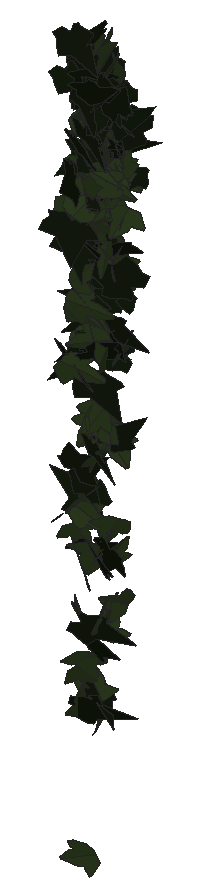
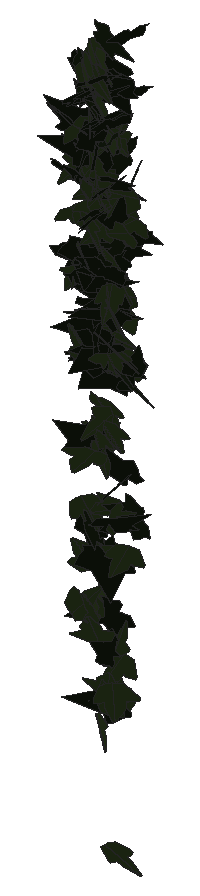
# SketchUp Ruby script. Lengths in inches.
U = 1.inch
M = Sketchup.active_model
def pt(a) = Geom::Point3d.new(a.map { |v| v * U })
def face(e, loops, mat)
  f = e.add_face(loops[0].map { |a| pt(a) })
  loops[1..].each { |l| e.add_face(l.map { |a| pt(a) }).erase! }
  f.material = f.back_material = mat if mat
  f
end
# faces: each face lists its corners as indices into pts; further lists are holes
def faces(e, pts, list, mat = nil) = list.each { |f| face(e, (f[0].is_a?(Array) ? f : [f]).map { |l| l.map { |i| pts[i] } }, mat) }
# xy, xz, yz: faces in a plane at the given z, y or x. An outline is a flat list of corners, or four numbers for a rectangle; further outlines are holes
def ring(l) = l.size == 4 ? [[l[0], l[1]], [l[2], l[1]], [l[2], l[3]], [l[0], l[3]]] : l.each_slice(2).to_a
def flat(e, list, mat, &to3) = list.each { |f| face(e, (f[0].is_a?(Array) ? f : [f]).map { |l| ring(l).map { |u, v| to3.(u, v) } }, mat) }
def xy(e, z, list, mat = nil) = flat(e, list, mat) { |x, y| [x, y, z] }
def xz(e, y, list, mat = nil) = flat(e, list, mat) { |x, z| [x, y, z] }
def yz(e, x, list, mat = nil) = flat(e, list, mat) { |y, z| [x, y, z] }
def lines(e, pts, list) = list.each { |a, b| e.add_line(pt(pts[a]), pt(pts[b])) }
# prism: a flat outline (further loops are holes) pulled along v
def prism(e, loops, v, mat = nil)
  f = face(e, loops, mat); d = Geom::Vector3d.new(v.map { |x| x * U })
  f.pushpull(f.normal.samedirection?(d) ? d.length : -d.length)
end
def box(e, o, s, mat = nil) = prism(e, [[o, [o[0] + s[0], o[1], o[2]], [o[0] + s[0], o[1] + s[1], o[2]], [o[0], o[1] + s[1], o[2]]]], [0, 0, s[2]], mat)
def at(x, y, z, deg = 0) = Geom::Transformation.translation(pt([x, y, z])) * Geom::Transformation.rotation(ORIGIN, Z_AXIS, deg.degrees)
def axes(o, x, y, z) = Geom::Transformation.new([*x, 0, *y, 0, *z, 0, *pt(o).to_a, 1])
def part(name) = M.definitions.add(name)
# library, detail: a bought-in or finely detailed component or shape, given as its bounding box
def library(name, o, s) = part(name).tap { |d| box(d.entities, o, s) }
def detail(e, o, s) = box(e.add_group.entities, o, s)
def put(e, d, t, mat = nil) = e.add_instance(d, t).tap { |i| i.material = mat if mat }
def group(e, t, mat = nil) = e.add_group.tap { |g| g.transformation = t; g.material = mat if mat }.entities
root = M.entities
M.materials.add("1026 AP 7946 SUNNY SIDE UP").color = [254, 231, 186]
M.materials.add("efeu1").color = [18, 25, 13]
M.materials.add("efeu2").color = [43, 57, 29]
c1 = part("ivyleaf_10")
p = [[0,0.5,-0.03],[-0.0625,2.02,-0.43],[-0.19,2.01,-0.46],[-0.54,1.05,-0.29],[-0.52,0.625,-0.18],[-0.83,0.76,-0.28],
  [-1.16,0.64,-0.33],[-1.15,0.33,-0.24],[-0.77,-0.39,0.02],[-0.3,-0.51,0.16],[0.04,-0.48,0.23],[-0.02,2.01,-0.4375],
  [-0.06,2.01,-0.43],[0.04,-0.49,0.23],[0.67,-0.49,0.14],[1.38,0.36,-0.2],[1.375,0.51,-0.24],[0.81,0.65,-0.19],
  [0.62,0.59,-0.15],[0.6,1.09,-0.28],[0.5,1.23,-0.31]]
faces(c1.entities,p,[[0,1,2,3,4,5,6,7,8,9,10],[11,12,0,13,14,15,16,17,18,19,20]],"efeu2")
c2 = part("ivyleaf_9")
p = [[1.54,2.16,1.25],[1.36,2.04,1.19],[-0.21,0.99,0.68],[-0.71,1.11,0.82],[-0.85,0.86,0.67],[-0.8,0.17,0.21],
  [-0.9,-0.01,0.1],[-0.67,-0.16,-0.02],[-0.08,-0.08,-0.05],[-0.03,-0.6,-0.4],[0.65,-0.88,-0.66],[0.83,-0.6,-0.49],
  [1.29,-0.42,-0.43],[1.8125,-0.07,-0.26],[1.21,0.44,0.15]]
faces(c2.entities,p,[[0,1,2,3,4,5,6,7,8,9,10,11,12,13,14]],"efeu1")
put(root,c1,axes([112.32,212.58,262.16],[0.2763,-0.17067,-0.05977],[0.08284,-0.02746,0.25162],[-0.27056,-0.18269,0.016]),"1026 AP 7946 SUNNY SIDE UP")
put(root,c2,axes([112.64,212.18,261],[-0.35335,0.1338,-0.06385],[0.06641,-0.05128,-0.26879],[-0.22268,-0.22761,0.02116]),"1026 AP 7946 SUNNY SIDE UP")
put(root,c1,axes([112.42,212.25,257.27],[-0.22363,-0.16972,-0.11593],[0.13077,0.0756,-0.22725],[0.29137,-0.16419,0.01301]),"1026 AP 7946 SUNNY SIDE UP")
put(root,c1,axes([112.52,212.29,255.31],[-0.24576,0.18393,0.0036],[0.01054,0.00248,0.24858],[0.28905,0.1563,-0.006]),"1026 AP 7946 SUNNY SIDE UP")
put(root,c1,axes([112.53,212.48,254.42],[-0.26293,-0.21485,0.00041],[0.01833,-0.01112,-0.28005],[0.33734,-0.16685,0.01554]),"1026 AP 7946 SUNNY SIDE UP")
put(root,c2,axes([112.67,212.58,265.125],[-0.37632,-0.06247,0.0594],[-0.07698,-0.04082,-0.2536],[0.10975,-0.24285,0.02579]),"1026 AP 7946 SUNNY SIDE UP")
put(root,c2,axes([112.74,212.43,257.79],[-0.29869,-0.19911,-0.04621],[-0.05273,-0.02843,0.28329],[-0.31617,0.19284,-0.00359]),"1026 AP 7946 SUNNY SIDE UP")
put(root,c1,axes([112.34,212.1875,264.2],[-0.27957,-0.08913,-0.13707],[0.24883,-0.07137,-0.16966],[0.0341,-0.20996,0.11426]),"1026 AP 7946 SUNNY SIDE UP")
put(root,c1,axes([112.56,212.46,266.07],[0.03135,-0.22524,0.12427],[0.00019,-0.12227,-0.23346],[0.40271,0.01759,-0.00956]),"1026 AP 7946 SUNNY SIDE UP")
put(root,c2,axes([112.33,212.16,266.99],[0.09061,-0.19392,-0.16045],[0.07592,0.16449,-0.19301],[0.38255,0.01328,0.07631]),"1026 AP 7946 SUNNY SIDE UP")
put(root,c2,axes([112.48,211.77,257.76],[-0.06386,0.25255,-0.09168],[-0.0318,0.08831,0.26397],[0.42059,0.04503,0.00604]),"1026 AP 7946 SUNNY SIDE UP")
put(root,c2,axes([112.51,212.09,264.69],[-0.03269,-0.0761,0.28244],[-0.09868,-0.26734,-0.08279],[0.43705,-0.06605,0.00243]),"1026 AP 7946 SUNNY SIDE UP")
put(root,c2,axes([112.51,212.01,263.88],[-0.26999,-0.16735,-0.12115],[0.14648,0.07132,-0.24625],[0.28536,-0.19494,0.01178]),"1026 AP 7946 SUNNY SIDE UP")
put(root,c2,axes([112.77,212.51,261.75],[-0.34185,0.11338,-0.00493],[-0.00847,-0.02204,-0.2517],[-0.17828,-0.21635,0.02143]),"1026 AP 7946 SUNNY SIDE UP")
put(root,c1,axes([112.56,212.48,262.77],[-0.14162,-0.25149,-0.10523],[0.09043,0.08596,-0.27362],[0.41626,-0.10424,0.02364]),"1026 AP 7946 SUNNY SIDE UP")
put(root,c1,axes([112.27,212.35,264.83],[-0.0931,-0.0054,-0.26878],[0.39706,-0.06857,-0.05798],[-0.10334,-0.25857,0.01937]),"1026 AP 7946 SUNNY SIDE UP")
put(root,c2,axes([112.44,212.58,266.46],[0.04423,-0.2333,-0.12414],[-0.00425,0.11959,-0.24115],[0.41191,0.02629,0.01084]),"1026 AP 7946 SUNNY SIDE UP")
put(root,c1,axes([112.41,212.44,266.1],[0.07251,-0.14138,0.2086],[0.26726,-0.1323,-0.13529],[0.28314,0.16109,0.07427]),"1026 AP 7946 SUNNY SIDE UP")
put(root,c1,axes([112.34,212.38,264.0625],[0.23882,0.01083,0.20798],[0.31655,-0.03048,-0.15457],[0.02817,0.25074,-0.02628]),"1026 AP 7946 SUNNY SIDE UP")
put(root,c1,axes([112.66,212.3,257.89],[0.0368,0.03694,-0.25423],[-0.13133,-0.23263,-0.04536],[-0.37007,0.08623,-0.00918]),"1026 AP 7946 SUNNY SIDE UP")
put(root,c1,axes([112.59,212.35,264.58],[-0.07442,0.22567,-0.06463],[0.0126,-0.06372,-0.23786],[-0.36864,-0.04773,0.00492]),"1026 AP 7946 SUNNY SIDE UP")
put(root,c1,axes([112.65,212.4,264.57],[0.30029,0.12402,-0.07462],[-0.09595,-0.04031,-0.23482],[-0.20505,0.20048,0.00061]),"1026 AP 7946 SUNNY SIDE UP")
put(root,c1,axes([112.55,212.625,262.64],[-0.03571,0.10642,-0.25194],[0.06017,-0.24221,-0.11339],[-0.41591,-0.04418,0.00523]),"1026 AP 7946 SUNNY SIDE UP")
put(root,c2,axes([112.43,212.18,265.57],[0.30095,-0.21064,0.01925],[-0.00065,-0.02718,-0.29274],[0.33269,0.1905,-0.01798]),"1026 AP 7946 SUNNY SIDE UP")
put(root,c1,axes([112.65,212.43,261.37],[0.29796,0.14273,-0.06151],[-0.05722,-0.05195,-0.24391],[-0.23696,0.19202,-0.01845]),"1026 AP 7946 SUNNY SIDE UP")
put(root,c2,axes([112.39,212.06,260.9],[0.14027,-0.16506,0.24365],[0.13509,-0.22214,-0.19364],[0.43418,0.12244,-0.01847]),"1026 AP 7946 SUNNY SIDE UP")
put(root,c1,axes([112.54,212.3,266.01],[0.14169,0.20034,0.1309],[0.10074,0.10905,-0.22534],[-0.35818,0.10992,-0.0116]),"1026 AP 7946 SUNNY SIDE UP")
put(root,c2,axes([112.55,212.35,262.46],[0.02897,0.10758,-0.25264],[-0.0118,0.24653,0.11201],[0.42179,-0.00049,0.02048]),"1026 AP 7946 SUNNY SIDE UP")
put(root,c2,axes([112.62,212.16,263.49],[-0.17884,-0.2304,-0.06982],[0.05918,0.0555,-0.26422],[0.37238,-0.11947,0.00846]),"1026 AP 7946 SUNNY SIDE UP")
put(root,c2,axes([112.47,212.51,264.37],[-0.01172,-0.06513,0.25169],[0.1762,-0.22036,-0.0582],[0.35702,0.10662,0.03698]),"1026 AP 7946 SUNNY SIDE UP")
put(root,c2,axes([112.55,212.56,265.04],[0.08673,-0.24778,-0.04562],[-0.0048,0.04323,-0.26118],[0.39537,0.05488,0.00683]),"1026 AP 7946 SUNNY SIDE UP")
put(root,c2,axes([112.59,211.92,267.98],[0.08654,-0.23035,-0.15185],[-0.03314,0.145,-0.24286],[0.42762,0.05785,0.01191]),"1026 AP 7946 SUNNY SIDE UP")
put(root,c1,axes([112.69,212.52,263.6],[0.32967,-0.13557,0.05425],[0.0548,-0.04425,-0.25681],[0.22247,0.21179,-0.01713]),"1026 AP 7946 SUNNY SIDE UP")
put(root,c1,axes([112.61,212.07,264.14],[0.26202,0.07095,-0.16182],[0.18111,0.11742,0.18074],[0.20238,-0.19692,0.04776]),"1026 AP 7946 SUNNY SIDE UP")
put(root,c1,axes([112.75,212.55,267.6],[0.20593,-0.22152,0.04877],[0.01978,-0.04894,-0.26501],[0.35605,0.13084,-0.01348]),"1026 AP 7946 SUNNY SIDE UP")
put(root,c2,axes([112.95,212.375,261.3],[-0.0124,0.01839,-0.27797],[-0.09809,-0.26289,-0.01811],[-0.41396,0.06175,0.01262]),"1026 AP 7946 SUNNY SIDE UP")
put(root,c2,axes([112.9,212.26,267.06],[0.08514,0.13614,-0.21514],[-0.08235,-0.20353,-0.15131],[-0.38428,0.07378,-0.01524]),"1026 AP 7946 SUNNY SIDE UP")
put(root,c2,axes([112.85,212.25,257.03],[0.22671,0.19448,-0.12512],[-0.09876,-0.10583,-0.24976],[-0.3477,0.15687,-0.01064]),"1026 AP 7946 SUNNY SIDE UP")
put(root,c1,axes([113.08,212.52,267.28],[-0.272,0.06176,0.22464],[-0.349,0.00713,-0.18373],[-0.06939,-0.27797,0.04349]),"1026 AP 7946 SUNNY SIDE UP")
put(root,c2,axes([112.76,212.6,265.875],[-0.1826,-0.13166,0.20436],[0.02255,-0.22488,-0.14588],[0.37467,-0.05063,0.10838]),"1026 AP 7946 SUNNY SIDE UP")
put(root,c2,axes([112.77,212.32,262.7],[0.3352,0.11882,-0.07713],[-0.08569,-0.05676,-0.25073],[-0.20414,0.21893,-0.0214]),"1026 AP 7946 SUNNY SIDE UP")
put(root,c2,axes([112.57,212.44,263.54],[0.14607,-0.18149,0.13892],[0.12398,-0.11181,-0.21005],[0.33424,0.12079,0.0172]),"1026 AP 7946 SUNNY SIDE UP")
put(root,c2,axes([112.85,212.73,267.22],[-0.23439,-0.18305,0.10121],[-0.04473,-0.10305,-0.24034],[0.32436,-0.14648,0.03999]),"1026 AP 7946 SUNNY SIDE UP")
put(root,c2,axes([112.68,212.32,266.92],[-0.24552,0.05136,0.22624],[0.32449,-0.07434,0.16886],[0.14195,0.25876,0.0053]),"1026 AP 7946 SUNNY SIDE UP")
put(root,c2,axes([112.58,212.2,263.39],[0.38865,-0.09854,0.03463],[0.0358,-0.03481,-0.27323],[0.16004,0.24708,-0.02298]),"1026 AP 7946 SUNNY SIDE UP")
put(root,c1,axes([113.03,211.85,250.64],[0.22812,-0.0603,-0.19784],[-0.28836,0.05695,-0.1611],[0.12921,0.23356,-0.01026]),"1026 AP 7946 SUNNY SIDE UP")
put(root,c2,axes([113.13,212.46,262.26],[-0.25336,0.01359,0.19712],[-0.30141,-0.01779,-0.16516],[0.00769,-0.24946,0.02104]),"1026 AP 7946 SUNNY SIDE UP")
put(root,c2,axes([112.95,212.31,268],[-0.29052,0.10303,-0.15225],[0.13213,-0.13886,-0.20795],[-0.25144,-0.19202,0.06665]),"1026 AP 7946 SUNNY SIDE UP")
put(root,c2,axes([112.7,212.07,258.53],[0.14013,-0.21846,-0.08117],[-0.04752,0.07143,-0.24265],[0.3614,0.0941,-0.00043]),"1026 AP 7946 SUNNY SIDE UP")
put(root,c2,axes([112.92,212.25,261.15],[0.06011,-0.16385,0.19178],[0.01813,0.19025,0.17033],[-0.39063,-0.01638,0.03742]),"1026 AP 7946 SUNNY SIDE UP")
put(root,c2,axes([112.625,211.98,258.68],[-0.07446,0.06318,0.24526],[0.27491,-0.16162,0.07919],[0.27203,0.18063,-0.0129]),"1026 AP 7946 SUNNY SIDE UP")
put(root,c1,axes([112.82,212.48,266.57],[0.19781,-0.21835,0.10618],[0.06042,-0.09805,-0.25975],[0.37568,0.13074,-0.01413]),"1026 AP 7946 SUNNY SIDE UP")
put(root,c2,axes([113.17,212.51,262.74],[-0.08357,0.04744,0.27061],[-0.41785,0.01284,-0.05776],[-0.03488,-0.26743,0.04361]),"1026 AP 7946 SUNNY SIDE UP")
put(root,c2,axes([112.67,212.58,263.33],[-0.11573,-0.1264,-0.21153],[0.243,0.1391,-0.14498],[0.28976,-0.16714,0.0371]),"1026 AP 7946 SUNNY SIDE UP")
put(root,c1,axes([112.69,212.03,262.1],[-0.27476,-0.05924,-0.18908],[0.29266,0.01136,-0.18661],[0.0775,-0.25292,0.03435]),"1026 AP 7946 SUNNY SIDE UP")
put(root,c1,axes([112.81,212.5625,265.09],[-0.36957,0.04222,0.09246],[0.14129,-0.00564,0.24577],[0.06522,0.25144,-0.0085]),"1026 AP 7946 SUNNY SIDE UP")
put(root,c2,axes([112.77,212.52,266.35],[-0.04784,-0.25611,0.00167],[0.00337,-0.00335,-0.26571],[0.40273,-0.0304,0.00242]),"1026 AP 7946 SUNNY SIDE UP")
put(root,c1,axes([112.65,211.78,261.01],[-0.17673,-0.10261,-0.24683],[0.35786,0.08726,-0.14834],[0.19801,-0.24929,0.04779]),"1026 AP 7946 SUNNY SIDE UP")
put(root,c1,axes([112.9,211.96,253.72],[-0.15032,-0.25931,-0.10103],[-0.0637,-0.08798,0.2841],[-0.43042,0.10358,-0.00676]),"1026 AP 7946 SUNNY SIDE UP")
put(root,c2,axes([113,211.85,256.49],[0.02553,-0.15099,0.20711],[-0.02113,0.20151,0.15754],[-0.39585,-0.0205,0.00495]),"1026 AP 7946 SUNNY SIDE UP")
put(root,c1,axes([113.03,212.16,256.99],[-0.36302,-0.13243,0.08801],[-0.09922,-0.06262,-0.27364],[0.22778,-0.23834,0.02107]),"1026 AP 7946 SUNNY SIDE UP")
put(root,c2,axes([112.9,212.12,262.04],[0.2513,-0.2063,0.04837],[-0.02623,0.04784,0.26862],[-0.33206,-0.1599,0.01539]),"1026 AP 7946 SUNNY SIDE UP")
put(root,c2,axes([112.78,212.6875,265.7],[0.05222,-0.1086,-0.23475],[0.28823,-0.14677,0.099],[-0.2716,-0.17664,0.05993]),"1026 AP 7946 SUNNY SIDE UP")
put(root,c1,axes([112.75,211.875,262.81],[0.26692,-0.1597,-0.09879],[0.14606,-0.0385,0.23746],[-0.25304,-0.19068,0.03286]),"1026 AP 7946 SUNNY SIDE UP")
put(root,c1,axes([113.17,212.09,261.57],[-0.13629,-0.03798,0.2463],[-0.28068,-0.16184,-0.09402],[0.25761,-0.19643,0.02787]),"1026 AP 7946 SUNNY SIDE UP")
put(root,c1,axes([112.97,212.14,259.69],[0.38834,-0.07504,-0.06318],[-0.10347,-0.00818,-0.26459],[0.1113,0.25424,-0.02554]),"1026 AP 7946 SUNNY SIDE UP")
put(root,c1,axes([112.99,212.48,267.77],[0.06995,-0.26071,-0.03214],[-0.01936,0.02803,-0.27219],[0.41214,0.04557,-0.00733]),"1026 AP 7946 SUNNY SIDE UP")
put(root,c2,axes([112.64,212.46,265.65],[0.28927,-0.04611,-0.18964],[0.2965,0.01896,0.18963],[-0.02975,-0.25937,0.046]),"1026 AP 7946 SUNNY SIDE UP")
put(root,c1,axes([112.9,211.79,254.62],[-0.16271,-0.18226,-0.1891],[0.1529,0.15459,-0.21492],[0.37567,-0.14186,0.00557]),"1026 AP 7946 SUNNY SIDE UP")
put(root,c1,axes([112.76,212.67,264.96],[0.1069,-0.07348,0.24964],[0.28925,-0.15872,-0.1035],[0.27454,0.19584,0.01184]),"1026 AP 7946 SUNNY SIDE UP")
put(root,c2,axes([112.8125,212.54,264.35],[0.11063,-0.23294,-0.0668],[-0.03084,0.06043,-0.25033],[0.3784,0.07303,-0.00088]),"1026 AP 7946 SUNNY SIDE UP")
put(root,c2,axes([112.83,212.0625,266.66],[0.03008,-0.24627,0.06307],[0.00957,-0.06233,-0.25483],[0.39944,0.02004,0.00136]),"1026 AP 7946 SUNNY SIDE UP")
put(root,c2,axes([112.86,212.49,264.41],[0.0454,-0.2375,-0.06441],[-0.01086,0.06078,-0.24611],[0.38547,0.02968,0.00065]),"1026 AP 7946 SUNNY SIDE UP")
put(root,c1,axes([112.95,212.34,264.98],[0.21719,-0.18767,0.10846],[0.07435,-0.09687,-0.23994],[0.33094,0.14493,-0.01728]),"1026 AP 7946 SUNNY SIDE UP")
put(root,c1,axes([113,212.04,254.06],[0.38554,0.03148,0.02966],[-0.04933,0.02072,0.25355],[0.04519,-0.24598,0.02368]),"1026 AP 7946 SUNNY SIDE UP")
put(root,c1,axes([113.04,212.52,264.98],[-0.05997,-0.1598,0.2045],[0.02831,-0.2028,-0.16506],[0.40082,-0.00958,0.04225]),"1026 AP 7946 SUNNY SIDE UP")
put(root,c1,axes([112.93,212.28,263.95],[-0.1332,-0.12812,-0.18731],[0.17548,0.14291,-0.15711],[0.30145,-0.1398,0.00869]),"1026 AP 7946 SUNNY SIDE UP")
put(root,c1,axes([112.98,212.1,259.84],[0.00006,0.12926,0.27294],[-0.01638,0.26404,-0.13153],[-0.4622,-0.00934,0.00469]),"1026 AP 7946 SUNNY SIDE UP")
put(root,c1,axes([113.04,212.51,267.57],[0.0309,-0.22724,0.13554],[0.02851,-0.13175,-0.23567],[0.41292,0.0261,0.00613]),"1026 AP 7946 SUNNY SIDE UP")
put(root,c1,axes([112.98,212.28,264.72],[0.01185,-0.02089,0.29138],[-0.01335,0.28291,0.0234],[-0.44593,-0.00903,0.00704]),"1026 AP 7946 SUNNY SIDE UP")
put(root,c2,axes([112.92,212.2,261.38],[0.20668,0.19532,0.16736],[0.17457,0.11898,-0.24086],[-0.35807,0.17074,-0.02083]),"1026 AP 7946 SUNNY SIDE UP")
put(root,c1,axes([113.09,212.18,253.46],[0.09696,-0.21994,-0.09048],[-0.04812,0.08129,-0.23473],[0.36854,0.06848,-0.00685]),"1026 AP 7946 SUNNY SIDE UP")
put(root,c2,axes([113.13,212.73,262.31],[-0.28365,-0.12462,0.10616],[-0.05899,-0.11892,-0.21503],[0.24806,-0.17078,0.07025]),"1026 AP 7946 SUNNY SIDE UP")
put(root,c1,axes([113.17,212.49,264.1],[0.25062,-0.14907,-0.14124],[-0.14851,0.09841,-0.22416],[0.28069,0.18516,0.00751]),"1026 AP 7946 SUNNY SIDE UP")
put(root,c1,axes([113.3,212.26,265.07],[0.13594,-0.10717,-0.25847],[-0.29249,0.16851,-0.13954],[0.31262,0.20426,-0.01816]),"1026 AP 7946 SUNNY SIDE UP")
put(root,c2,axes([112.91,212.39,266.89],[0.02557,-0.26139,-0.08793],[0.02819,0.08485,-0.26834],[0.43072,0.00996,0.02279]),"1026 AP 7946 SUNNY SIDE UP")
put(root,c2,axes([112.85,211.99,265.98],[0.14766,-0.23332,0.08269],[0.05102,-0.07489,-0.25953],[0.38529,0.09933,0.00268]),"1026 AP 7946 SUNNY SIDE UP")
put(root,c1,axes([113.11,212.39,266.25],[0.07254,-0.22436,-0.1264],[-0.00169,0.12322,-0.23426],[0.40113,0.0411,0.02187]),"1026 AP 7946 SUNNY SIDE UP")
put(root,c2,axes([112.81,212.69,265.99],[0.09173,-0.12131,0.21859],[0.18702,-0.17729,-0.1387],[0.33681,0.13148,0.01748]),"1026 AP 7946 SUNNY SIDE UP")
put(root,c1,axes([113.11,212.53,267.29],[0.09856,-0.25443,-0.00032],[0.00096,-0.00101,-0.26995],[0.40007,0.06268,0.00073]),"1026 AP 7946 SUNNY SIDE UP")
put(root,c2,axes([112.8,212.18,254.97],[0.11448,-0.06692,0.23241],[0.20078,-0.18759,-0.10071],[0.31147,0.14552,-0.0205]),"1026 AP 7946 SUNNY SIDE UP")
put(root,c1,axes([112.77,211.83,262.35],[-0.04663,-0.0243,-0.27243],[0.41464,-0.03302,-0.02755],[-0.04758,-0.26391,0.02695]),"1026 AP 7946 SUNNY SIDE UP")
put(root,c2,axes([113.25,211.91,267.04],[0.13231,0.15885,-0.20878],[-0.18153,-0.16837,-0.1855],[-0.36317,0.14203,0.01666]),"1026 AP 7946 SUNNY SIDE UP")
put(root,c1,axes([112.85,212.36,264.32],[0.20743,-0.12757,-0.20087],[0.26942,-0.09753,0.18528],[-0.24689,-0.21361,0.03341]),"1026 AP 7946 SUNNY SIDE UP")
put(root,c1,axes([113.14,212.02,260.06],[0.37368,-0.10989,-0.05061],[-0.08471,-0.00141,-0.26865],[0.16881,0.24254,-0.02278]),"1026 AP 7946 SUNNY SIDE UP")
put(root,c1,axes([113.03,212.37,265.42],[-0.10562,0.16322,-0.20774],[0.06328,-0.20018,-0.18108],[-0.40414,-0.074,0.02594]),"1026 AP 7946 SUNNY SIDE UP")
put(root,c1,axes([113.16,212.07,259.17],[-0.01498,-0.28605,-0.00426],[0.00177,0.00248,-0.29484],[0.44981,-0.00954,0.00102]),"1026 AP 7946 SUNNY SIDE UP")
put(root,c1,axes([112.87,211.89,257.9],[0.17738,0.07498,0.20068],[0.26839,0.09347,-0.13865],[-0.18783,0.20438,-0.00861]),"1026 AP 7946 SUNNY SIDE UP")
put(root,c2,axes([113.15,212.39,263.43],[0.2196,0.20048,-0.06469],[-0.0392,-0.06042,-0.25167],[-0.32855,0.14121,-0.01321]),"1026 AP 7946 SUNNY SIDE UP")
put(root,c1,axes([113.11,212.26,259.5625],[0.35459,-0.09909,0.04331],[0.04763,-0.03657,-0.25305],[0.16278,0.22656,-0.02029]),"1026 AP 7946 SUNNY SIDE UP")
put(root,c2,axes([113.39,212.46,261.19],[-0.16189,-0.21276,-0.09909],[-0.06382,-0.08587,0.24299],[-0.36076,0.11067,0.00148]),"1026 AP 7946 SUNNY SIDE UP")
put(root,c1,axes([113.26,212.48,264.2],[-0.02951,-0.06949,0.24323],[-0.05583,-0.23394,-0.07509],[0.38354,-0.0394,0.00778]),"1026 AP 7946 SUNNY SIDE UP")
put(root,c2,axes([113.39,212.55,266.53],[-0.17532,0.0427,0.236],[-0.30305,-0.15923,-0.06707],[0.20528,-0.19861,0.10254]),"1026 AP 7946 SUNNY SIDE UP")
put(root,c1,axes([113.11,212.24,255.26],[0.33034,0.10498,-0.0688],[0.07699,0.05198,0.24102],[0.1804,-0.21442,0.02311]),"1026 AP 7946 SUNNY SIDE UP")
put(root,c1,axes([113.22,212.54,263.43],[0.18162,-0.21654,-0.00869],[-0.02874,-0.0016,-0.25224],[0.33946,0.11572,-0.01671]),"1026 AP 7946 SUNNY SIDE UP")
put(root,c2,axes([113,211.99,259.38],[0.20319,-0.21582,0.00639],[-0.01196,-0.0132,-0.25886],[0.33935,0.12876,-0.01295]),"1026 AP 7946 SUNNY SIDE UP")
put(root,c2,axes([113.17,212.37,266.63],[-0.15907,-0.22825,0.07243],[-0.03767,-0.06768,-0.25754],[0.37426,-0.10383,0.00486]),"1026 AP 7946 SUNNY SIDE UP")
put(root,c2,axes([112.88,211.81,253.74],[0.24099,0.04046,0.2207],[0.33931,0.0072,-0.16057],[-0.04634,0.26313,-0.02796]),"1026 AP 7946 SUNNY SIDE UP")
put(root,c1,axes([113.21,212.46,264.88],[0.10894,-0.22724,0.07759],[0.01311,-0.07741,-0.24478],[0.37685,0.06838,-0.01391]),"1026 AP 7946 SUNNY SIDE UP")
put(root,c1,axes([113.03,212.5,259.23],[0.24916,0.17716,0.11396],[0.14013,0.06684,-0.24361],[-0.29609,0.18071,-0.0194]),"1026 AP 7946 SUNNY SIDE UP")
put(root,c2,axes([113.06,212.13,254.12],[0.08616,-0.24444,-0.00888],[-0.00995,0.006,-0.25798],[0.38439,0.05495,-0.00468]),"1026 AP 7946 SUNNY SIDE UP")
put(root,c2,axes([113.05,211.89,261.375],[0.25943,0.16015,0.14293],[0.18352,0.0767,-0.23529],[-0.27697,0.20084,-0.02202]),"1026 AP 7946 SUNNY SIDE UP")
put(root,c2,axes([113,212.11,256.86],[0.05238,-0.1067,0.22953],[0.12531,-0.2088,-0.11619],[0.36857,0.08616,0.00689]),"1026 AP 7946 SUNNY SIDE UP")
put(root,c2,axes([113.43,212.11,266.45],[-0.10379,0.20861,0.14425],[-0.08036,0.12935,-0.22449],[-0.38574,-0.08308,0.00796]),"1026 AP 7946 SUNNY SIDE UP")
put(root,c2,axes([113.33,212.28,261.37],[0.13394,-0.1484,0.18801],[-0.09133,0.17573,0.17536],[-0.35947,-0.09994,0.0255]),"1026 AP 7946 SUNNY SIDE UP")
put(root,c2,axes([113.25,212.37,265.73],[0.24874,-0.09952,-0.20107],[-0.28514,0.07438,-0.1906],[0.1919,0.23951,-0.02258]),"1026 AP 7946 SUNNY SIDE UP")
put(root,c2,axes([113.04,212.03,260.72],[-0.13949,-0.10809,-0.2339],[0.27707,0.14413,-0.14116],[0.28085,-0.19587,0.02308]),"1026 AP 7946 SUNNY SIDE UP")
put(root,c1,axes([113.3,212.58,266.03],[0.11745,0.17134,-0.18079],[-0.15062,-0.14959,-0.19229],[-0.35622,0.11975,0.02169]),"1026 AP 7946 SUNNY SIDE UP")
put(root,c2,axes([113.01,211.77,255.61],[0.06467,0.02429,-0.25584],[0.20771,0.21157,0.04507],[0.33311,-0.13664,0.02156]),"1026 AP 7946 SUNNY SIDE UP")
put(root,c1,axes([113.16,212.18,263.49],[0.27571,-0.1274,0.14547],[0.14831,-0.10964,-0.22208],[0.26066,0.19715,-0.02751]),"1026 AP 7946 SUNNY SIDE UP")
put(root,c1,axes([113.24,212.12,255.65],[0.10436,-0.22111,0.09404],[-0.03151,0.09057,0.23827],[-0.37558,-0.06904,0.00614]),"1026 AP 7946 SUNNY SIDE UP")
put(root,c1,axes([113.24,212.3,256.83],[-0.07669,-0.22927,0.09718],[0.02584,0.09427,0.24201],[-0.38976,0.05136,-0.00308]),"1026 AP 7946 SUNNY SIDE UP")
put(root,c1,axes([113.4,212.46,255.86],[-0.07823,-0.1147,-0.25567],[-0.18393,-0.21834,0.12718],[-0.38753,0.12678,-0.00875]),"1026 AP 7946 SUNNY SIDE UP")
put(root,c1,axes([113.32,211.75,255.65],[0.14811,-0.18162,0.15472],[-0.09324,0.13941,0.21137],[-0.35972,-0.11092,0.00891]),"1026 AP 7946 SUNNY SIDE UP")
put(root,c2,axes([113.34,212.2,257.55],[-0.21129,0.08097,-0.19782],[0.22591,-0.13026,-0.16053],[-0.23829,-0.19529,0.02322]),"1026 AP 7946 SUNNY SIDE UP")
put(root,c2,axes([113.05,212.29,261.8],[0.04994,-0.02362,-0.24881],[0.285,0.16408,0.00899],[0.25342,-0.17987,0.03893]),"1026 AP 7946 SUNNY SIDE UP")
put(root,c1,axes([113.21,212.48,263.02],[0.13566,0.20822,0.11523],[0.08405,0.0975,-0.23135],[-0.36112,0.10091,-0.01056]),"1026 AP 7946 SUNNY SIDE UP")
put(root,c1,axes([113.37,212.3,263.07],[-0.05501,0.18767,0.1807],[-0.09314,0.16526,-0.19454],[-0.39185,-0.06562,0.02087]),"1026 AP 7946 SUNNY SIDE UP")
put(root,c2,axes([113.0625,212.39,265.53],[0.12518,0.02448,0.25985],[0.3893,0.04821,-0.08509],[-0.08399,0.25994,-0.0071]),"1026 AP 7946 SUNNY SIDE UP")
put(root,c1,axes([113.39,211.76,261.37],[0.0147,0.06879,-0.2538],[0.01208,0.24673,0.07261],[0.40261,-0.00991,0.00709]),"1026 AP 7946 SUNNY SIDE UP")
put(root,c1,axes([113.47,212.16,264.91],[0.04136,0.18003,0.18854],[-0.09155,-0.17395,0.18492],[0.39197,-0.05962,0.02329]),"1026 AP 7946 SUNNY SIDE UP")
put(root,c2,axes([113.5,211.87,266.95],[-0.01742,0.25779,0.09736],[0.00073,0.09314,-0.26524],[-0.43094,-0.01026,-0.00439]),"1026 AP 7946 SUNNY SIDE UP")
put(root,c1,axes([113.15,212.03,265.01],[-0.23406,-0.08921,-0.23867],[0.34842,0.07277,-0.1755],[0.17438,-0.26514,0.03029]),"1026 AP 7946 SUNNY SIDE UP")
put(root,c2,axes([113.63,211.96,266.7],[0.02894,0.01863,0.29897],[-0.20637,0.2599,-0.00709],[-0.40785,-0.13019,0.02481]),"1026 AP 7946 SUNNY SIDE UP")
put(root,c2,axes([113.75,212.17,262.91],[-0.11673,0.03781,0.28589],[-0.42975,0.05191,-0.08236],[-0.09465,-0.28233,0.02141]),"1026 AP 7946 SUNNY SIDE UP")
put(root,c2,axes([113.26,212.26,259.36],[-0.07667,-0.00132,0.25166],[0.35432,0.09598,0.04743],[-0.14838,0.22988,-0.01678]),"1026 AP 7946 SUNNY SIDE UP")
put(root,c1,axes([113.45,212.46,264.19],[0.23787,0.15478,-0.12393],[-0.12361,-0.09251,-0.22337],[-0.28329,0.17033,-0.00659]),"1026 AP 7946 SUNNY SIDE UP")
put(root,c1,axes([113.54,212.04,257.82],[-0.22775,-0.18562,0.08852],[-0.0615,-0.07952,-0.24239],[0.31641,-0.14907,0.01661]),"1026 AP 7946 SUNNY SIDE UP")
put(root,c2,axes([113.78,212.47,266.07],[-0.30758,0.15738,0.13897],[-0.18823,0.06415,-0.25727],[-0.26496,-0.22827,0.02144]),"1026 AP 7946 SUNNY SIDE UP")
put(root,c2,axes([113.54,212.62,265.12],[-0.36065,-0.02852,-0.0751],[0.11847,-0.02104,-0.23638],[0.03252,-0.2397,0.02825]),"1026 AP 7946 SUNNY SIDE UP")
put(root,c2,axes([113.26,212.35,265.99],[-0.12131,0.01557,0.26726],[0.40835,0.0123,0.0789],[-0.01159,0.27029,-0.0174]),"1026 AP 7946 SUNNY SIDE UP")
put(root,c1,axes([113.41,212.3,261.21],[0.11033,-0.25815,0.05587],[-0.00078,0.05751,0.27553],[-0.41525,-0.06869,0.01433]),"1026 AP 7946 SUNNY SIDE UP")
put(root,c2,axes([113.55,211.83,257.35],[0.24824,-0.02357,-0.20514],[-0.31501,-0.01302,-0.16223],[0.0069,0.25368,-0.02589]),"1026 AP 7946 SUNNY SIDE UP")
put(root,c1,axes([113.37,212.26,265.16],[0.06094,0.20294,0.20474],[0.06924,0.19269,-0.21165],[-0.43995,0.05844,-0.00495]),"1026 AP 7946 SUNNY SIDE UP")
put(root,c1,axes([113.53,212.32,265.22],[0.30309,-0.13731,0.13488],[-0.14914,0.09319,0.24363],[-0.25935,-0.21405,0.01753]),"1026 AP 7946 SUNNY SIDE UP")
